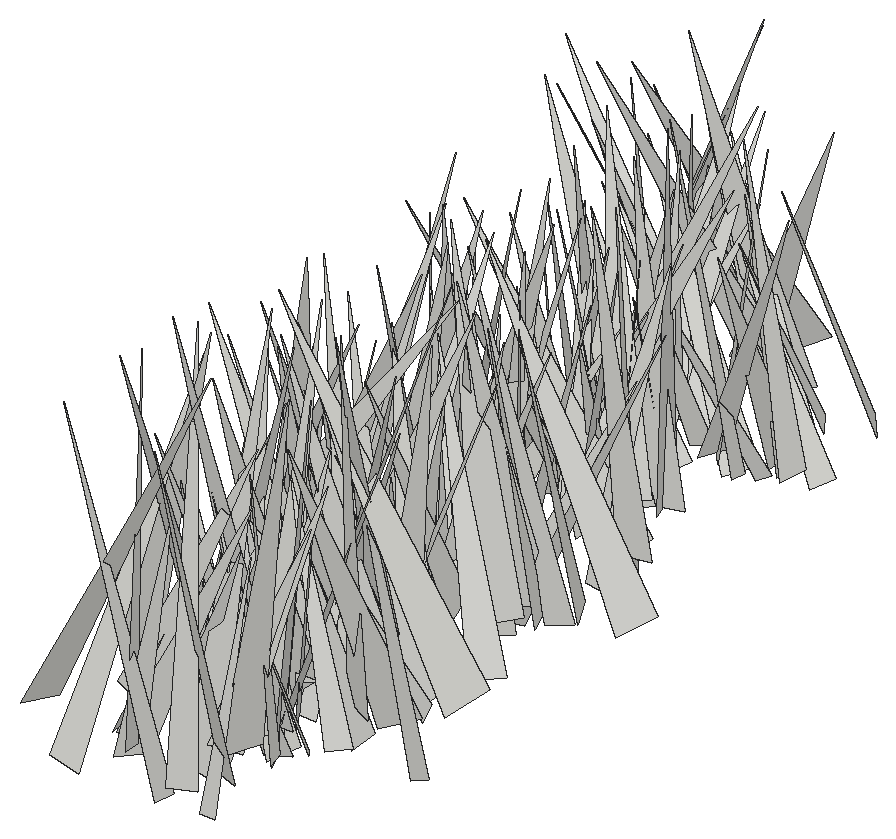
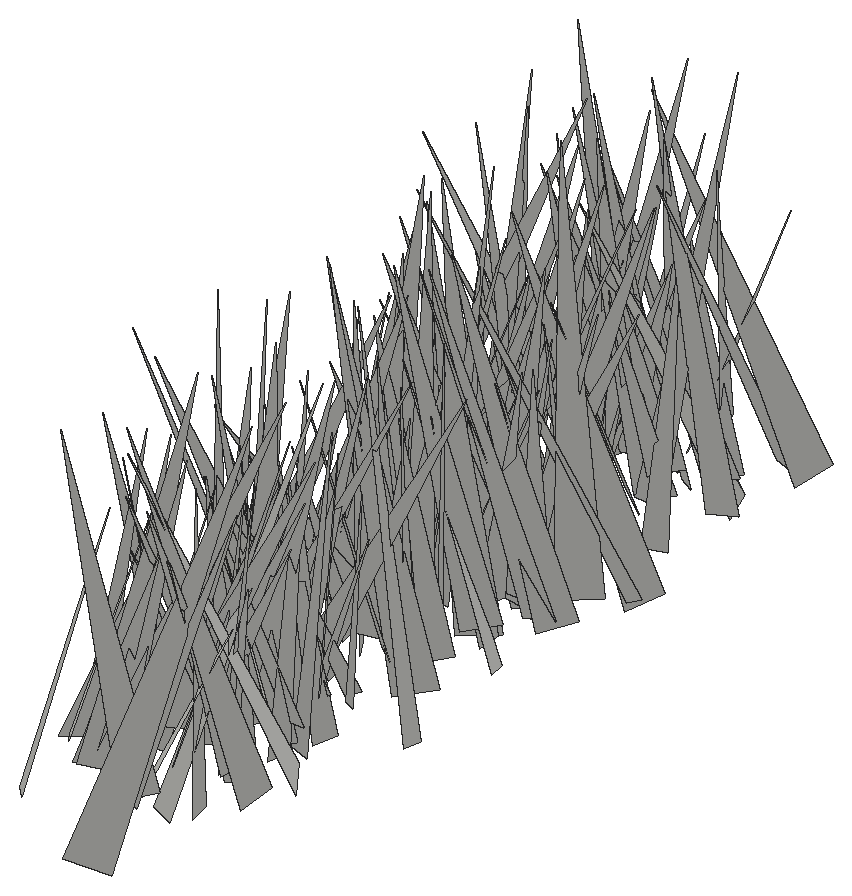
# SketchUp Ruby script. Lengths in inches.
U = 1.inch
M = Sketchup.active_model
def pt(a) = Geom::Point3d.new(a.map { |v| v * U })
def face(e, loops, mat)
  f = e.add_face(loops[0].map { |a| pt(a) })
  loops[1..].each { |l| e.add_face(l.map { |a| pt(a) }).erase! }
  f.material = f.back_material = mat if mat
  f
end
# faces: each face lists its corners as indices into pts; further lists are holes
def faces(e, pts, list, mat = nil) = list.each { |f| face(e, (f[0].is_a?(Array) ? f : [f]).map { |l| l.map { |i| pts[i] } }, mat) }
# xy, xz, yz: faces in a plane at the given z, y or x. An outline is a flat list of corners, or four numbers for a rectangle; further outlines are holes
def ring(l) = l.size == 4 ? [[l[0], l[1]], [l[2], l[1]], [l[2], l[3]], [l[0], l[3]]] : l.each_slice(2).to_a
def flat(e, list, mat, &to3) = list.each { |f| face(e, (f[0].is_a?(Array) ? f : [f]).map { |l| ring(l).map { |u, v| to3.(u, v) } }, mat) }
def xy(e, z, list, mat = nil) = flat(e, list, mat) { |x, y| [x, y, z] }
def xz(e, y, list, mat = nil) = flat(e, list, mat) { |x, z| [x, y, z] }
def yz(e, x, list, mat = nil) = flat(e, list, mat) { |y, z| [x, y, z] }
def lines(e, pts, list) = list.each { |a, b| e.add_line(pt(pts[a]), pt(pts[b])) }
# prism: a flat outline (further loops are holes) pulled along v
def prism(e, loops, v, mat = nil)
  f = face(e, loops, mat); d = Geom::Vector3d.new(v.map { |x| x * U })
  f.pushpull(f.normal.samedirection?(d) ? d.length : -d.length)
end
def box(e, o, s, mat = nil) = prism(e, [[o, [o[0] + s[0], o[1], o[2]], [o[0] + s[0], o[1] + s[1], o[2]], [o[0], o[1] + s[1], o[2]]]], [0, 0, s[2]], mat)
def at(x, y, z, deg = 0) = Geom::Transformation.translation(pt([x, y, z])) * Geom::Transformation.rotation(ORIGIN, Z_AXIS, deg.degrees)
def axes(o, x, y, z) = Geom::Transformation.new([*x, 0, *y, 0, *z, 0, *pt(o).to_a, 1])
def part(name) = M.definitions.add(name)
# library, detail: a bought-in or finely detailed component or shape, given as its bounding box
def library(name, o, s) = part(name).tap { |d| box(d.entities, o, s) }
def detail(e, o, s) = box(e.add_group.entities, o, s)
def put(e, d, t, mat = nil) = e.add_instance(d, t).tap { |i| i.material = mat if mat }
def group(e, t, mat = nil) = e.add_group.tap { |g| g.transformation = t; g.material = mat if mat }.entities
root = M.entities
c1 = part("fur_instance\#9")
p = [[0.8125,0,1.79],[0.67,-0.02,1.48],[0,-0.11,0],[0,0.11,0]]
faces(c1.entities,p,[[0,1,2,3]])
put(root,c1,axes([153.55,108.53,-27.1],[-3.32572,-4.76152,1.64129],[-5.0351,3.09772,-1.21581],[-0.11678,2.03921,5.67929]))
put(root,c1,axes([151.43,107.83,-28.22],[-6.70794,-1.60484,0.19836],[-1.59675,6.44001,-1.8942],[-0.25542,1.88735,6.63204]))
put(root,c1,axes([153.3125,107.73,-28.22],[1.45734,4.18221,0.34787],[4.02467,-1.49715,1.13854],[-1.18907,0.05834,4.28]))
put(root,c1,axes([148.6875,109.36,-28.22],[4.06657,-2.17936,1.39694],[-2.40276,-4.14574,0.52683],[-0.9632,1.14071,4.58356]))
put(root,c1,axes([145.28,108.9375,-27.1],[7.55011,-1.58138,0.22082],[-1.59514,-7.42262,1.38345],[0.0711,1.39915,7.58887]))
put(root,c1,axes([152.63,110.35,-27.1],[7.05562,-2.47543,1.6862],[-2.53392,-7.23407,-0.01726],[-1.59697,0.54154,7.47725]))
put(root,c1,axes([152.75,107.08,-27.1],[1.27817,7.72916,0.81529],[7.27012,-1.48113,2.64386],[-2.74773,-0.32349,7.37453]))
put(root,c1,axes([149.71,108.25,-27.1],[-6.21182,-1.68937,2.27799],[-2.42044,6.01654,-2.13837],[1.47806,2.75267,6.07191]))
put(root,c1,axes([148.25,110.21,-28.22],[2.73482,-5.11249,1.4467],[-5.08402,-2.04521,2.38319],[1.54377,2.32148,5.28557]))
put(root,c1,axes([147.43,107.55,-28.22],[2.14003,7.20036,0.0672],[7.19519,-2.14104,0.27303],[-0.28086,0.01341,7.50668]))
put(root,c1,axes([151.27,110.4,-28.22],[-0.77235,4.89048,2.70767],[4.92537,1.88806,-2.00519],[2.64368,-2.08884,4.52687]))
put(root,c1,axes([152.19,110.1,-27.1],[3.72107,-3.56028,1.90501],[-4.03778,-3.30047,1.71878],[-0.03061,2.5656,4.85467]))
put(root,c1,axes([153.92,110.5625,-27.1],[-4.56501,-1.69942,1.47091],[-1.97129,4.62695,-0.77219],[1.07964,1.26263,4.80947]))
put(root,c1,axes([149.29,111.69,-27.1],[1.54528,-3.8993,0.59524],[-3.77652,-1.27799,1.43226],[1.13873,1.05307,3.94222]))
put(root,c1,axes([147.49,111.03,-27.1],[1.43912,5.66343,2.07225],[5.60003,-0.46439,-2.61988],[2.23794,-2.47985,5.22319]))
put(root,c1,axes([149.64,110.57,-28.22],[1.92341,3.31368,0.82854],[3.39872,-1.95136,-0.08567],[-0.34002,-0.7604,3.83049]))
put(root,c1,axes([148.56,114.02,-27.1],[-2.04467,-7.63412,0.65301],[-7.56547,2.11851,1.07815],[1.21235,0.345,7.82931]))
put(root,c1,axes([152.45,112.36,-27.1],[-1.50167,-7.67594,2.08534],[-7.92089,1.24921,-1.10571],[-0.72669,2.24569,7.7429]))
put(root,c1,axes([152.58,112.41,-28.22],[-1.01411,-6.0227,1.51425],[-5.97973,0.53295,-1.88497],[-1.67593,1.7428,5.80932]))
put(root,c1,axes([154.5,111.61,-27.1],[-3.00148,-2.27694,0.1564],[-2.20162,2.82047,-1.1898],[-0.60148,1.03841,3.57459]))
put(root,c1,axes([151.32,109.875,-28.22],[1.82525,7.99707,1.79582],[8.16577,-1.93273,0.30716],[-0.70587,-1.67961,8.19697]))
put(root,c1,axes([152.65,112.6,-28.22],[4.1746,-2.61988,2.8232],[-2.37692,-5.02847,-1.15163],[-3.03059,0.33503,4.79215]))
put(root,c1,axes([151.42,111.74,-27.1],[-2.68831,3.38264,1.06218],[3.54497,2.54168,0.8778],[-0.06058,-1.37662,4.23069]))
put(root,c1,axes([150.42,110.86,-28.22],[5.15508,0.33774,1.32609],[0.02228,-5.18864,1.23487],[-1.36825,1.188,5.01637]))
put(root,c1,axes([146.02,113.1,-27.1],[-0.11111,-7.60969,2.49454],[-7.52897,0.94928,2.56048],[2.72852,2.30953,7.16685]))
put(root,c1,axes([147.23,110.78,-28.22],[6.4283,2.09347,0.22673],[2.03253,-6.35917,1.08941],[-0.55031,0.96716,6.67224]))
put(root,c1,axes([150.71,110.44,-28.22],[-5.03448,1.97141,0.87824],[1.57247,4.87743,-1.93439],[1.47821,1.52579,5.04882]))
put(root,c1,axes([152.58,112.35,-28.22],[5.91365,2.78735,2.33328],[2.94924,-6.28377,0.03183],[-2.12497,-0.96423,6.53755]))
put(root,c1,axes([151.46,111.56,-27.1],[-5.91196,3.62871,1.99788],[3.48429,6.23911,-1.02156],[2.24027,-0.12769,6.86114]))
put(root,c1,axes([151.6875,113.63,-27.1],[-3.71371,1.13934,1.58672],[1.47505,3.87017,0.67337],[1.28063,-1.15373,3.82574]))
put(root,c1,axes([150.93,111.29,-28.22],[-5.01986,0.40192,1.5189],[-0.17545,4.90978,-1.87904],[1.56135,1.84392,4.67223]))
put(root,c1,axes([149.36,113.05,-27.1],[7.16515,0.1083,1.44204],[0.09788,-7.3087,0.06254],[-1.44279,0.042,7.1657]))
put(root,c1,axes([155.14,112.38,-27.1],[-1.55107,4.41542,0.77186],[4.34501,1.28043,1.40671],[-1.10114,-1.16708,4.46351]))
put(root,c1,axes([147.5625,114.97,-28.22],[0.34868,-5.31048,0.36463],[-5.26358,-0.28954,0.81646],[0.79301,0.41316,5.25892]))
put(root,c1,axes([151.18,115.66,-28.22],[2.6009,-7.25193,0.96085],[-7.2129,-2.71231,-0.94648],[-1.21974,0.57558,7.64587]))
put(root,c1,axes([151.65,114.56,-28.22],[4.17117,1.8451,1.43695],[2.27213,-3.89306,-1.59669],[-0.55375,-2.07548,4.27243]))
put(root,c1,axes([154.36,116.59,-28.22],[3.73251,-5.71066,0.85994],[-5.41751,-3.81707,-1.83396],[-2.00044,-0.31799,6.57114]))
put(root,c1,axes([148.45,113.29,-27.1],[-1.13275,3.97734,1.11963],[3.98013,1.3621,-0.81189],[1.10966,-0.82546,4.05502]))
put(root,c1,axes([152.58,111.68,-27.1],[-6.84761,2.51212,1.52779],[1.98246,6.80446,-2.30302],[2.17135,1.70976,6.92074]))
put(root,c1,axes([153.93,114.9,-27.1],[2.87262,5.81566,3.24646],[6.49078,-3.23727,0.05584],[-1.49368,-2.88298,6.48619]))
put(root,c1,axes([154.2,114.87,-28.22],[-7.29173,-1.24054,0.1592],[-1.24954,7.26646,-0.60898],[0.05425,0.6271,7.37139]))
put(root,c1,axes([151.49,115.35,-27.1],[1.53479,-3.08573,1.52348],[-3.30012,-1.79268,-0.30636],[-0.97569,1.2095,3.43271]))
put(root,c1,axes([149.94,114.93,-28.22],[0.29151,4.89673,1.62599],[5.06271,0.04273,-1.03633],[0.99541,-1.65136,4.79468]))
put(root,c1,axes([152.48,112.89,-27.1],[7.12213,3.78972,1.00867],[3.4176,-7.02352,2.25704],[-1.92338,1.55314,7.74548]))
put(root,c1,axes([156.5,117.49,-27.1],[-7.92246,2.32052,1.49756],[2.68865,7.5204,2.57051],[0.63138,-2.90715,7.84491]))
put(root,c1,axes([152.32,118.54,-27.1],[-1.3783,-7.92591,0.91068],[-7.76861,1.54372,1.6777],[1.81604,0.58822,7.86798]))
put(root,c1,axes([157.26,114.04,-28.22],[-6.80362,-1.51626,0.05987],[-1.39466,6.13985,-2.9915],[-0.59797,2.93174,6.29597]))
put(root,c1,axes([150.99,116.89,-27.1],[-5.87282,3.13064,1.60123],[3.47052,5.66214,1.65846],[0.56601,-2.23474,6.44519]))
put(root,c1,axes([153.12,117.17,-27.1],[-6.41083,1.14128,1.69671],[1.48537,6.43646,1.28286],[1.40536,-1.59673,6.38401]))
put(root,c1,axes([150.27,115.89,-28.22],[-3.29969,1.99263,1.18367],[2.06312,3.46364,-0.07948],[1.05601,-0.54058,3.85386]))
put(root,c1,axes([154.64,117.7,-28.22],[-3.89152,-1.38284,0.09587],[-1.31779,3.77936,1.02238],[0.42995,-0.93252,4.00136]))
put(root,c1,axes([150.27,118.06,-28.22],[7.85727,-0.11013,0.63762],[0.0287,-7.70188,-1.68396],[-0.64642,-1.6806,7.67549]))
put(root,c1,axes([151.7,114.98,-28.22],[0.7,4.04155,0.09862],[4.02713,-0.70587,0.34334],[-0.35517,-0.03822,4.08733]))
put(root,c1,axes([150.79,117.21,-27.1],[5.32067,-0.59583,0.38531],[-0.58759,-5.33383,-0.13414],[-0.39777,-0.09079,5.35224]))
put(root,c1,axes([149.07,114.3,-27.1],[2.7978,5.22834,0.27095],[4.99402,-2.75746,1.64099],[-1.57121,0.54549,5.69828]))
put(root,c1,axes([150.0625,115.9,-28.22],[0.28645,5.00767,1.03913],[5.08565,-0.389,0.47271],[-0.54104,-1.00525,4.99354]))
put(root,c1,axes([151.7,117.05,-28.22],[-4.53112,4.00144,0.54603],[3.94801,4.21612,1.86503],[-0.85024,-1.74745,5.75015]))
put(root,c1,axes([148.94,119.4,-28.22],[1.68994,-6.65431,0.98946],[-6.7239,-1.70391,0.02495],[-0.21912,0.96522,6.8655]))
put(root,c1,axes([151.57,119.33,-28.22],[-1.24664,-7.42641,1.30497],[-7.49381,1.07378,-1.04811],[-0.83512,1.45053,7.45702]))
put(root,c1,axes([153.03,118.31,-27.1],[-4.85785,0.78834,1.37895],[1.02249,4.94749,0.77364],[1.21552,-1.0112,4.86021]))
put(root,c1,axes([154.17,118.51,-28.22],[-7.15146,0.58689,0.88826],[0.71619,7.11549,1.06478],[0.78773,-1.14116,7.09606]))
put(root,c1,axes([145.48,118.08,-28.22],[7.07032,-2.50038,0.22823],[-2.5064,-6.98854,1.08245],[0.14815,1.09629,7.42089]))
put(root,c1,axes([151.49,119.78,-27.1],[1.84889,-3.8875,0.07331],[-3.87281,-1.83403,0.41727],[0.34554,0.24513,4.2845]))
put(root,c1,axes([152.54,118.85,-27.1],[5.43979,-3.16023,1.66658],[-3.30816,-5.60189,0.17546],[-1.34931,0.9938,6.28869]))
put(root,c1,axes([148.35,118.48,-28.22],[-2.09497,-3.98677,2.51489],[-4.46346,2.56262,0.34425],[1.51546,2.03632,4.49052]))
put(root,c1,axes([146.16,120.89,-27.1],[5.23004,-6.31048,0.45418],[-6.32662,-5.22094,0.31214],[-0.04891,0.54893,8.19012]))
put(root,c1,axes([152.39,116.93,-28.22],[-7.44461,1.33123,0.56849],[1.18187,7.30967,-1.63995],[0.83578,1.52121,7.38274]))
put(root,c1,axes([149.02,120.9,-28.22],[-0.33805,-5.61743,0.95415],[-5.65981,0.22074,-0.70569],[-0.6576,0.9879,5.58317]))
put(root,c1,axes([151.75,121.38,-27.1],[-3.32799,-2.15223,0.18164],[-2.02775,3.22824,1.09879],[0.74386,-0.82886,3.80792]))
put(root,c1,axes([152.36,122.26,-27.1],[-5.45284,-1.57742,1.94379],[-0.6971,5.43147,2.45217],[2.40429,-2.00271,5.11943]))
put(root,c1,axes([144.63,119.77,-27.1],[4.68753,6.76488,0.69054],[6.04009,-3.75687,-4.19721],[3.12373,-2.88717,7.07954]))
put(root,c1,axes([149.41,120.37,-27.1],[1.51862,3.68557,2.40948],[4.21899,-1.94756,0.31991],[-1.2606,-2.07817,3.97332]))
put(root,c1,axes([152.75,119.74,-28.22],[3.04965,-4.5466,3.26672],[-5.09549,-3.79519,-0.52522],[-2.31926,2.35973,5.44941]))
put(root,c1,axes([151.41,121.52,-28.22],[-4.06839,-1.50308,0.30492],[-1.46625,4.06536,0.47647],[0.44983,-0.34301,4.31092]))
put(root,c1,axes([151.27,119.51,-28.22],[4.3993,3.63087,0.47155],[3.65139,-4.40515,-0.14642],[-0.27004,-0.41338,5.70225]))
put(root,c1,axes([148.82,120.04,-27.1],[-2.21571,3.96483,0.99922],[4.07213,2.24229,0.13245],[0.36886,-0.93805,4.54001]))
put(root,c1,axes([148.46,120.84,-28.22],[1.17731,-6.81979,2.88625],[-6.91612,0.0321,2.89694],[2.64712,3.11697,6.28517]))
put(root,c1,axes([150.86,121.81,-27.1],[4.29298,-1.68508,0.76366],[-1.68331,-4.35833,-0.1541],[-0.76754,0.13347,4.60928]))
put(root,c1,axes([147.9375,119.79,-28.22],[3.62964,3.56201,0.97293],[3.43547,-3.75775,0.94107],[-1.35352,0.01415,4.99765]))
put(root,c1,axes([149.92,124.04,-27.1],[-3.16207,-7.07316,1.24758],[-6.76016,3.39142,2.09364],[2.42619,0.2311,7.45956]))
put(root,c1,axes([154.75,120.74,-28.22],[-3.19469,4.99874,1.10839],[5.10889,3.02549,1.08057],[-0.33936,-1.5103,5.83317]))
put(root,c1,axes([153.87,122.41,-27.1],[-5.4764,4.5647,2.90915],[5.14181,5.68019,0.76664],[1.69155,-2.48788,7.08799]))
put(root,c1,axes([149.68,121.46,-28.22],[-5.43325,1.77797,0.85582],[1.73658,5.49897,-0.39929],[0.93695,0.1182,5.7028]))
put(root,c1,axes([145.53,122.9,-27.1],[5.33015,-4.46349,0.382],[-4.4244,-5.15196,1.5366],[0.7024,1.41905,6.78027]))
put(root,c1,axes([150.16,120.52,-27.1],[-2.57926,6.41675,1.59968],[6.21683,2.93816,-1.76197],[2.25493,-0.76079,6.68751]))
put(root,c1,axes([153.04,123.2,-28.22],[-3.30956,4.62511,3.28339],[5.43338,3.67626,0.29816],[1.62808,-2.86687,5.67942]))
put(root,c1,axes([154.05,123.96,-27.1],[2.81422,-5.9892,1.8303],[-5.99838,-3.15452,-1.09945],[-1.79999,1.14839,6.52546]))
put(root,c1,axes([148.58,123.46,-28.22],[-1.94061,6.26278,4.61542],[7.19839,3.24975,-1.38302],[2.95087,-3.80883,6.40903]))
put(root,c1,axes([150.88,124.44,-27.1],[2.46673,-5.38252,0.46134],[-5.39282,-2.42347,0.55987],[0.31917,0.65147,5.89431]))
put(root,c1,axes([154.875,123.32,-27.1],[-4.89111,-2.11302,1.38613],[-2.21595,5.03778,-0.13961],[1.21481,0.68196,5.3262]))
put(root,c1,axes([151.18,123.12,-27.1],[4.40781,-2.35415,1.32075],[-2.57038,-4.43283,0.67704],[-0.82436,1.23418,4.95101]))
put(root,c1,axes([148.25,121.27,-27.1],[3.95249,6.61953,0.92655],[6.54498,-4.05132,1.02412],[-1.35642,-0.25967,7.64143]))
put(root,c1,axes([146.36,122.87,-27.1],[0.74046,6.81709,2.01452],[6.9144,-0.22063,-1.79488],[1.64984,-2.13492,6.61811]))
put(root,c1,axes([149.95,125.16,-27.1],[-0.40221,-7.56998,1.93164],[-7.73436,0.65878,0.97125],[1.10251,1.85984,7.51818]))
put(root,c1,axes([152.04,123.25,-27.1],[-4.34264,3.05124,0.46122],[3.07623,4.34339,0.23041],[0.24406,-0.45414,5.3024]))
put(root,c1,axes([155.55,123.56,-27.1],[-0.37721,6.24874,2.25952],[6.16262,-0.51732,2.45945],[-2.4848,-2.23161,5.75674]))
put(root,c1,axes([147.99,123.59,-28.22],[4.52049,-0.19473,1.20973],[-0.39564,-4.60837,0.73662],[-1.15967,0.81315,4.46432]))
put(root,c1,axes([151.23,123.35,-27.1],[4.54007,-1.04122,1.07478],[-1.33062,-4.37982,1.37772],[-0.68465,1.60765,4.44952]))
put(root,c1,axes([146.53,125.02,-28.22],[5.44749,2.02001,0.26599],[2.02291,-5.27178,-1.39377],[0.24298,-1.39796,5.64031]))
put(root,c1,axes([152.01,123.85,-28.22],[0.9151,5.15761,1.58711],[5.35443,-1.06795,0.38322],[-0.67079,-1.48856,5.22413]))
put(root,c1,axes([147.56,124.57,-27.1],[3.87683,-5.48097,2.21285],[-5.90731,-3.50163,1.67625],[0.20355,2.76859,6.50085]))
put(root,c1,axes([154.39,126.14,-28.22],[-4.88015,-2.78524,1.52655],[-2.68194,5.11285,0.7548],[1.7015,0.07051,5.5681]))
put(root,c1,axes([149.27,124.75,-28.22],[-5.47988,-2.79163,2.54101],[-3.31815,5.69792,-0.89593],[1.79996,2.00489,6.08438]))
put(root,c1,axes([152.01,124.23,-27.1],[-4.80614,1.67739,0.07303],[1.63862,4.73444,-0.90443],[0.36591,0.83033,5.00945]))
put(root,c1,axes([156.4,126.56,-28.22],[-6.88709,2.46248,0.81316],[2.58785,6.67518,1.70354],[0.16756,-1.88022,7.11293]))
put(root,c1,axes([151.17,126.76,-28.22],[4.52719,2.71843,2.25301],[3.1828,-4.72799,-0.69084],[-1.52829,-1.79378,5.23527]))
put(root,c1,axes([150.72,125.81,-28.22],[1.36969,7.27883,2.41401],[7.66649,-1.2409,-0.6083],[0.18385,-2.48268,7.38156]))
put(root,c1,axes([148.57,125.71,-28.22],[3.58302,-2.92408,2.58959],[-3.63927,-3.77537,0.77237],[-1.41842,2.30013,4.5598]))
put(root,c1,axes([150.25,127.43,-27.1],[0.10364,-5.95888,1.80759],[-6.13378,0.21397,1.05707],[1.07352,1.79787,5.86529]))
put(root,c1,axes([148.48,126.79,-28.22],[4.56446,-0.76979,0.5853],[-0.81155,-4.58493,0.29877],[-0.52586,0.39409,4.61927]))
put(root,c1,axes([149.42,126.3125,-27.1],[-4.67336,-1.61213,2.14084],[-2.03116,4.93814,-0.71533],[1.7483,1.42769,4.89159]))
put(root,c1,axes([147.71,128.04,-28.22],[4.04324,-6.81137,0.9787],[-6.74817,-3.70246,2.11055],[1.34718,1.89668,7.63467]))
put(root,c1,axes([153.12,124.24,-28.22],[5.35308,0.77922,1.1136],[0.09871,-4.73607,2.83947],[-1.35556,2.73224,4.60435]))
put(root,c1,axes([151.81,127.19,-27.1],[1.90499,3.12749,0.05078],[3.06447,-1.8542,-0.76405],[0.62675,-0.43991,3.5814]))
put(root,c1,axes([153.625,128.83,-28.22],[-3.79405,-1.81524,0.00607],[-1.81515,3.79397,0.03081],[0.01877,-0.02517,4.20582]))
put(root,c1,axes([154.67,128.58,-27.1],[-0.07394,-6.12578,2.47714],[-6.56947,-0.19789,-0.68546],[-0.70961,2.47033,6.08776]))
put(root,c1,axes([150.87,127.74,-27.1],[4.041,0.55824,1.1889],[0.26805,-4.11576,1.02147],[-1.28579,0.89645,3.94942]))
put(root,c1,axes([153.53,127.79,-28.22],[1.21689,3.56799,0.58582],[3.55761,-1.29191,0.47847],[-0.64586,-0.39367,3.73931]))
put(root,c1,axes([154.1,129.3,-28.22],[-4.17203,-5.0841,2.64194],[-5.48144,4.49304,-0.00972],[1.66784,2.04897,6.57676]))
put(root,c1,axes([149.01,128.08,-27.1],[-2.72966,-3.54913,3.67888],[-4.47058,3.67982,0.23296],[2.47878,2.72838,4.47136]))
put(root,c1,axes([150.45,130.74,-27.1],[-1.24481,-6.10899,0.55091],[-5.80958,0.99391,-2.10566],[-1.96776,0.93016,5.86818]))
put(root,c1,axes([145.52,130.99,-28.22],[7.53646,1.85279,1.2332],[2.16443,-7.11553,-2.53698],[-0.51849,-2.77277,7.33449]))
put(root,c1,axes([153.21,130.5625,-28.22],[-6.98354,0.71492,0.27676],[0.75932,6.7998,1.59491],[0.10557,-1.6153,6.83646]))
put(root,c1,axes([151.11,130.8,-28.22],[-6.05597,0.77226,2.0179],[1.21073,6.18666,1.26588],[1.78953,-1.57224,5.97233]))
put(root,c1,axes([151.07,131.42,-27.1],[3.64038,-1.44849,0.64201],[-1.22649,-3.59476,-1.15586],[-1.003,-0.8615,3.74359]))
put(root,c1,axes([151.11,130.24,-27.1],[4.61454,1.12705,1.27743],[1.23829,-4.75228,-0.2803],[-1.16993,-0.58453,4.7419]))
put(root,c1,axes([151.92,130.375,-27.1],[-1.54169,4.36128,2.00643],[4.43238,2.10262,-1.16464],[1.84406,-1.40768,4.47674]))
put(root,c1,axes([147.75,131.71,-27.1],[-1.86728,-3.21645,1.13397],[-3.16749,2.11482,0.78275],[1.26429,0.54787,3.63587]))
put(root,c1,axes([149.82,131.32,-28.22],[-3.79704,-0.30553,0.54536],[-0.26679,3.82814,0.28712],[0.56533,-0.2455,3.79848]))
put(root,c1,axes([149.16,131.58,-27.1],[-3.54566,-2.66431,1.6705],[-2.78653,3.82874,0.19209],[1.45754,0.83849,4.43096]))
put(root,c1,axes([150.44,130.44,-28.22],[-3.00951,3.51493,1.30262],[3.55292,3.20728,-0.44587],[1.1951,-0.68362,4.60577]))
put(root,c1,axes([148.16,130.98,-27.1],[1.07989,-3.22676,1.49499],[-3.22529,-0.23045,1.83235],[1.49815,1.82977,2.86716]))
put(root,c1,axes([149.51,130.12,-27.1],[3.96425,-0.56902,0.64503],[-0.79665,-3.57598,1.74151],[-0.32433,1.82859,3.60641]))
put(root,c1,axes([151.1,131.95,-27.1],[-4.28874,-2.62611,1.19653],[-2.76089,4.3576,-0.33198],[0.84,0.91449,5.01792]))
put(root,c1,axes([150.62,130.54,-27.1],[-4.55116,2.07867,0.64916],[1.93391,4.54938,-1.00919],[1.00113,0.66152,4.90056]))
put(root,c1,axes([152.11,131.44,-27.1],[-4.3858,5.26104,2.02142],[5.54364,4.48874,0.34523],[1.01623,-1.78118,6.84066]))
put(root,c1,axes([148.07,132.63,-28.22],[5.46664,-0.56538,0.68203],[-0.51758,-5.49848,-0.40957],[-0.71898,-0.34055,5.48051]))
put(root,c1,axes([151.73,129.49,-27.1],[-3.94545,3.07895,0.18102],[2.74281,3.63702,-2.08047],[1.41057,1.53994,4.55172]))
put(root,c1,axes([148.24,133.89,-28.22],[-2.50316,-5.2047,1.47138],[-5.2002,2.76171,0.92225],[1.48721,0.89649,5.70124]))
put(root,c1,axes([151.87,133.79,-28.22],[7.38345,1.68053,2.79244],[2.22073,-7.65548,-1.26461],[-2.38543,-1.92527,7.46594]))
put(root,c1,axes([151.1,132.11,-28.22],[-4.16278,-2.64249,2.71758],[-3.23685,4.57857,-0.50613],[1.97251,1.93665,4.90462]))
put(root,c1,axes([148.93,132.28,-27.1],[3.61026,-5.57217,1.81458],[-5.57053,-2.60139,3.09478],[1.81959,3.09184,5.87413]))
put(root,c1,axes([152.1,133.39,-28.22],[1.19646,-6.35488,2.45253],[-6.76034,-1.41301,-0.36331],[-0.83491,2.33448,6.45631]))
put(root,c1,axes([150.91,134.8,-27.1],[-2.708,-3.38854,1.07596],[-2.8715,2.88211,1.84961],[2.09627,-0.42942,3.92357]))
put(root,c1,axes([148.59,134.57,-28.22],[6.67439,0.3641,2.55328],[0.99441,-6.8993,-1.61558],[-2.3797,-1.86182,6.48614]))
put(root,c1,axes([149.13,133.65,-28.22],[0.1838,-6.38239,2.38865],[-6.46729,0.58989,2.0738],[2.14821,2.32195,6.03888]))
put(root,c1,axes([151,133.56,-28.22],[-7.00283,2.97011,1.6591],[3.21934,7.01289,1.03394],[1.10002,-1.61605,7.53606]))
put(root,c1,axes([152,134.19,-27.1],[-4.37284,2.10544,0.41102],[2.13916,4.20984,1.19366],[-0.16073,-1.25217,4.70423]))
put(root,c1,axes([148.8,134.64,-27.1],[3.81482,2.67004,0.71919],[2.75746,-3.58156,-1.32965],[0.20681,-1.49748,4.4625]))
put(root,c1,axes([151.71,134.01,-28.22],[-4.89428,-1.48699,1.50253],[-1.73277,4.99254,-0.70337],[1.21087,1.13406,5.0666]))
put(root,c1,axes([148.375,133.9375,-27.1],[4.07945,6.65627,1.20942],[6.56454,-3.55321,-2.58689],[1.63565,-2.3408,7.36585]))
put(root,c1,axes([149.08,135.78,-28.22],[0.94706,-3.59902,0.23008],[-3.53322,-0.8783,0.80484],[0.72266,0.42244,3.63347]))
put(root,c1,axes([151.45,134.51,-27.1],[-3.62089,2.64212,0.01483],[2.58278,3.53416,0.96476],[-0.55698,-0.78788,4.37731]))
put(root,c1,axes([151.77,133.26,-28.22],[-5.67085,1.89535,1.35099],[1.57668,5.74544,-1.44226],[1.71219,0.98676,5.80265]))
put(root,c1,axes([151.71,135.87,-27.1],[-0.61117,-4.98438,1.28841],[-4.9544,0.21679,-1.51148],[-1.3993,1.40945,4.78884]))
put(root,c1,axes([152.29,135.73,-27.1],[5.3173,-1.56529,0.48292],[-1.59322,-5.32309,0.28875],[-0.38078,0.41424,5.53538]))
put(root,c1,axes([149.72,136.82,-27.1],[0.99148,-3.49866,0.36174],[-3.47594,-0.91715,0.65665],[0.53788,0.52224,3.57665]))
put(root,c1,axes([153.12,138.45,-28.22],[5.27025,-2.47106,0.85487],[-2.00329,-5.05203,-2.25305],[-1.68041,-1.72721,5.36707]))
put(root,c1,axes([153.91,135.01,-27.1],[-5.8174,-1.77979,0.63377],[-1.88895,5.44209,-2.05595],[-0.03436,2.15114,5.72563]))
put(root,c1,axes([153.4,137.02,-28.22],[-1.12844,-4.06047,0.83548],[-3.60524,0.5338,-2.27512],[-2.04639,1.29864,3.54749]))
put(root,c1,axes([155.33,136.15,-27.1],[-5.94659,0.26274,1.16381],[0.1992,6.05181,-0.34844],[1.17635,0.30341,5.94219]))
put(root,c1,axes([149.81,138.56,-27.1],[-5.8383,-2.13052,1.19785],[-1.77007,5.82456,1.73238],[1.68547,-1.263,5.96857]))
put(root,c1,axes([150.07,135.64,-27.1],[-2.40389,3.30252,0.08348],[3.28439,2.37806,0.4999],[-0.35549,-0.36124,4.05406]))
put(root,c1,axes([152.52,135.64,-27.1],[3.86177,3.77021,1.4507],[3.73701,-4.09632,0.69796],[-1.5342,-0.48777,5.35169]))
put(root,c1,axes([149.22,140.3,-28.22],[-4.65731,-6.85842,0.0184],[-6.74044,4.58127,1.51895],[1.26677,-0.83835,8.14992]))
put(root,c1,axes([151.61,136.81,-27.1],[-6.06762,4.08752,0.30456],[4.00596,5.79855,1.98636],[-0.86766,-1.81261,7.04117]))
put(root,c1,axes([149.87,135.95,-28.22],[-6.10428,-1.79449,1.71008],[-2.20054,6.01533,-1.54278],[1.14113,2.0006,6.1727]))
put(root,c1,axes([152.52,136.9,-28.22],[-4.45803,3.98436,0.74293],[4.03358,4.25341,1.39275],[-0.39655,-1.52789,5.81458]))
put(root,c1,axes([155.17,137.92,-28.22],[-3.79672,1.89832,0.59417],[1.98792,3.66583,0.99077],[0.06937,-1.15319,4.1276]))
put(root,c1,axes([149.65,135.49,-28.22],[0.187,6.43803,0.46404],[6.40843,-0.12967,-0.78342],[0.77175,-0.48321,6.39292]))
put(root,c1,axes([151.7,140.23,-27.1],[1.64942,-7.33453,1.1804],[-6.83961,-1.97125,-2.69132],[-2.89974,0.47759,7.01946]))
put(root,c1,axes([148.56,136.97,-27.1],[0.79551,4.29487,0.6755],[4.10301,-0.51451,-1.56067],[1.4379,-0.90797,4.07959]))
put(root,c1,axes([153.92,139.56,-27.1],[-3.41692,-2.65793,0.41527],[-2.50813,3.39027,1.06197],[0.9728,-0.5949,4.19669]))
put(root,c1,axes([153.71,137.74,-28.22],[-4.7779,-0.84592,1.0787],[-0.97294,4.84801,-0.50762],[0.9657,0.69908,4.82558]))
put(root,c1,axes([147.12,135.4,-28.22],[6.47525,4.61232,0.40047],[4.47579,-6.41261,1.48613],[-1.18373,0.98374,7.80985]))
put(root,c1,axes([148.26,139.42,-28.22],[5.52429,1.58059,2.16664],[1.98524,-5.74559,-0.8703],[-1.80317,-1.48335,5.67966]))
put(root,c1,axes([151.67,140.625,-27.1],[3.93699,-6.31061,2.13001],[-6.14082,-4.39732,-1.67764],[-2.57895,0.83692,7.24632]))
put(root,c1,axes([148.37,136.8,-28.22],[-1.23708,6.4323,0.84499],[6.38548,1.35924,-0.99849],[1.14637,-0.62994,6.47363]))
put(root,c1,axes([148,137.79,-27.1],[4.12915,-1.39251,2.24683],[-2.1688,-4.1671,1.40312],[-1.51116,2.17563,4.12556]))
put(root,c1,axes([151.65,140.06,-27.1],[-5.54142,2.04017,2.02802],[2.50487,5.58649,1.22443],[1.41448,-1.90035,5.77671]))
put(root,c1,axes([150.91,139.03,-28.22],[-4.27231,-1.94809,0.06255],[-1.87913,4.07681,-1.37844],[-0.51754,1.27912,4.48861]))
put(root,c1,axes([146.11,138.94,-27.1],[7.40622,-0.19557,0.80001],[-0.28757,-7.3972,0.85392],[-0.77173,0.87956,7.35943]))
put(root,c1,axes([153.34,139.125,-28.22],[-3.45745,4.3845,0.64107],[4.38114,3.2607,1.32749],[-0.66366,-1.31634,5.42361]))
put(root,c1,axes([149.4,141.33,-27.1],[3.81645,-5.44593,0.15233],[-5.28758,-3.65777,1.70554],[1.31259,1.09964,6.42764]))
put(root,c1,axes([154.06,142.08,-28.22],[-3.97091,-3.72473,0.66515],[-3.58252,4.01146,1.07602],[1.21718,-0.34456,5.33703]))
put(root,c1,axes([149.63,141.73,-27.1],[-1.836,-5.36618,0.72675],[-5.38286,1.72484,-0.86298],[-0.59066,0.96126,5.60554]))
put(root,c1,axes([148.91,144.83,-28.22],[4.97759,-6.71856,0.2944],[-6.18791,-4.7191,-3.07278],[-2.63353,-1.61035,7.77647]))
